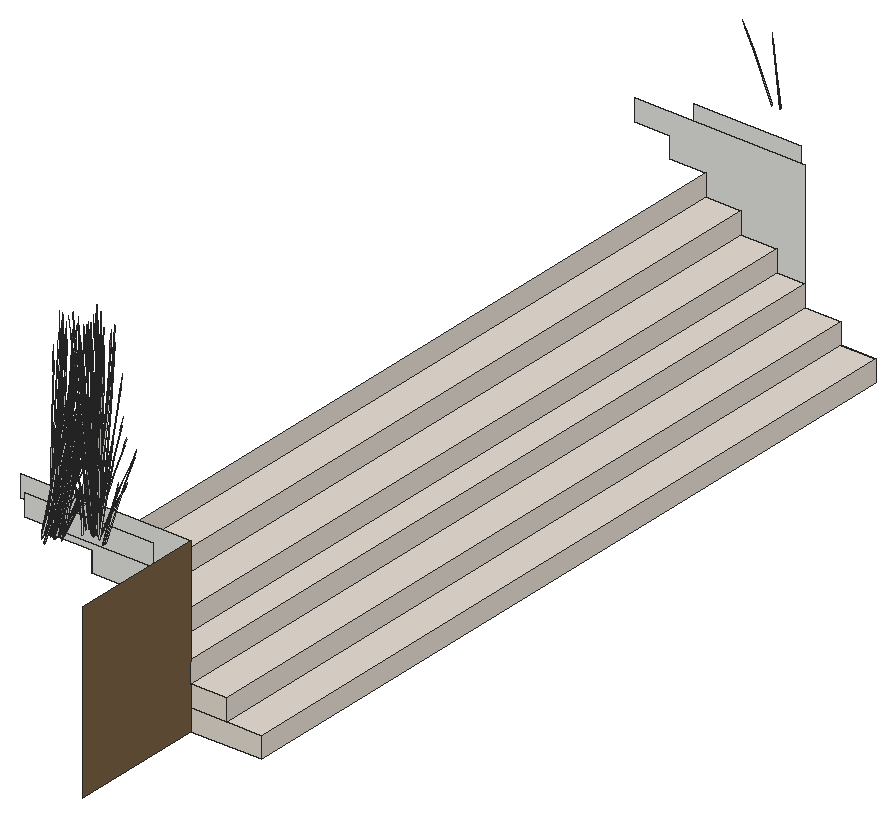
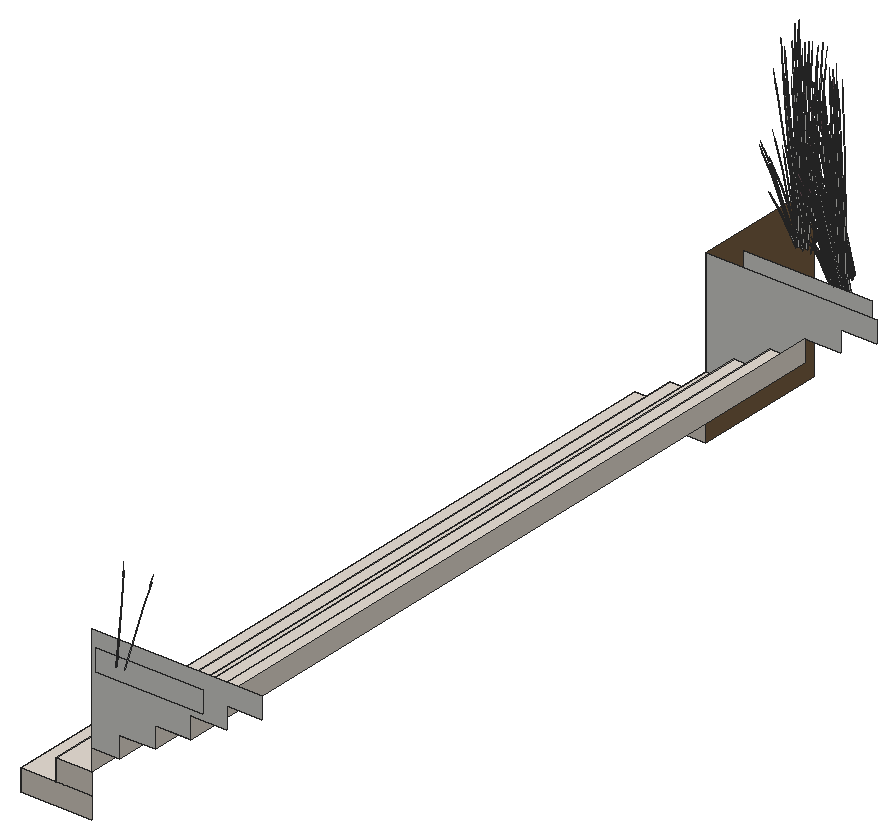
# SketchUp Ruby script. Lengths in inches.
U = 1.inch
M = Sketchup.active_model
def pt(a) = Geom::Point3d.new(a.map { |v| v * U })
def face(e, loops, mat)
  f = e.add_face(loops[0].map { |a| pt(a) })
  loops[1..].each { |l| e.add_face(l.map { |a| pt(a) }).erase! }
  f.material = f.back_material = mat if mat
  f
end
# faces: each face lists its corners as indices into pts; further lists are holes
def faces(e, pts, list, mat = nil) = list.each { |f| face(e, (f[0].is_a?(Array) ? f : [f]).map { |l| l.map { |i| pts[i] } }, mat) }
# xy, xz, yz: faces in a plane at the given z, y or x. An outline is a flat list of corners, or four numbers for a rectangle; further outlines are holes
def ring(l) = l.size == 4 ? [[l[0], l[1]], [l[2], l[1]], [l[2], l[3]], [l[0], l[3]]] : l.each_slice(2).to_a
def flat(e, list, mat, &to3) = list.each { |f| face(e, (f[0].is_a?(Array) ? f : [f]).map { |l| ring(l).map { |u, v| to3.(u, v) } }, mat) }
def xy(e, z, list, mat = nil) = flat(e, list, mat) { |x, y| [x, y, z] }
def xz(e, y, list, mat = nil) = flat(e, list, mat) { |x, z| [x, y, z] }
def yz(e, x, list, mat = nil) = flat(e, list, mat) { |y, z| [x, y, z] }
def lines(e, pts, list) = list.each { |a, b| e.add_line(pt(pts[a]), pt(pts[b])) }
# prism: a flat outline (further loops are holes) pulled along v
def prism(e, loops, v, mat = nil)
  f = face(e, loops, mat); d = Geom::Vector3d.new(v.map { |x| x * U })
  f.pushpull(f.normal.samedirection?(d) ? d.length : -d.length)
end
def box(e, o, s, mat = nil) = prism(e, [[o, [o[0] + s[0], o[1], o[2]], [o[0] + s[0], o[1] + s[1], o[2]], [o[0], o[1] + s[1], o[2]]]], [0, 0, s[2]], mat)
def at(x, y, z, deg = 0) = Geom::Transformation.translation(pt([x, y, z])) * Geom::Transformation.rotation(ORIGIN, Z_AXIS, deg.degrees)
def axes(o, x, y, z) = Geom::Transformation.new([*x, 0, *y, 0, *z, 0, *pt(o).to_a, 1])
def part(name) = M.definitions.add(name)
# library, detail: a bought-in or finely detailed component or shape, given as its bounding box
def library(name, o, s) = part(name).tap { |d| box(d.entities, o, s) }
def detail(e, o, s) = box(e.add_group.entities, o, s)
def put(e, d, t, mat = nil) = e.add_instance(d, t).tap { |i| i.material = mat if mat }
def group(e, t, mat = nil) = e.add_group.tap { |g| g.transformation = t; g.material = mat if mat }.entities
root = M.entities
M.materials.add("LightPink_Translucent").color = [144, 107, 117]
M.materials["LightPink_Translucent"].alpha = 0.75
M.materials.add("Marble_01_1K").color = [230, 221, 211]
M.materials.add("Soil_03_1K").color = [122, 96, 67]
c1 = part("blade")
p = [[2.15,0.21,22],[0,0.17,0],[0.09,0.45,0],[2.18,0.31,22],[2.29,0.31,22],[0.38,0.45,0],
  [2.48,0.24,33],[2.49,0.24,33],[2.48,0.22,33]]
faces(c1.entities,p,[[0,1,2,3],[4,5,2,3],[6,3,4,7],[8,0,3,6]])
c2 = part("seeds")
p = [[0.3,-0.1,1.38],[-0.01,-0.03,1.59],[-0.01,-0.03,0.03],[0.14,-0.07,-0.07],[0.29,-0.03,3],[0.15,0.01,3.11]]
faces(c2.entities,p,[[0,1,2,3],[1,0,4,5]],"LightPink_Translucent")
c3 = part("blade with seeds")
put(c3.entities,c1,at(0,0,0))
put(c3.entities,c2,axes([2.4,0.25,30.99],[1.5799,-0.05474,1.17369],[-0.12525,1.92788,0.29478],[-0.07173,-0.02425,1.56792]))
xy(root,6,[[362,46,372,262]],"Marble_01_1K")
xy(root,12,[[352,46,362,262]],"Marble_01_1K")
xy(root,18,[[344,46,352,262]],"Marble_01_1K")
xy(root,24,[[334,46,344,262]],"Marble_01_1K")
xy(root,30,[[324,46,334,262]],"Marble_01_1K")
xz(root,40,[[310,42,346,48]])
xz(root,46,[[344,18,344,24,334,24,334,30,324,30,324,36,314,36,314,42,304,42,304,48,352,48,352,18]])
xz(root,46,[[352,0,372,6],[352,6,362,12]],"Marble_01_1K")
xz(root,262,[[344,18,352,18,352,48,304,48,304,42,314,42,314,36,324,36,324,30,334,30,334,24,344,24]])
xz(root,262,[[352,0,372,6],[352,6,362,12]],"Marble_01_1K")
xz(root,268,[[316,42,346,48]])
yz(root,324,[[46,30,262,36]],"Marble_01_1K")
yz(root,334,[[46,24,262,30]],"Marble_01_1K")
yz(root,344,[[46,18,262,24]],"Marble_01_1K")
yz(root,352,[[46,12,262,18]],"Marble_01_1K")
yz(root,352,[[8,0,46,48]],"Soil_03_1K")
yz(root,362,[[46,6,262,12]],"Marble_01_1K")
yz(root,372,[[46,0,262,6]],"Marble_01_1K")
put(root,c3,axes([321.74,34.29,43.82],[0.34009,-0.2937,-0.55095],[0.42248,0.26632,-0.1446],[0.13628,-0.07327,1.21613]))
put(root,c3,axes([323.39,30.83,46.18],[-0.22948,0.24822,0.05682],[-0.32679,-0.14452,0.44729],[0.10565,0.07958,0.68204]))
put(root,c3,axes([324.1875,33.59,44.44],[-0.16818,0.19891,1.01491],[-0.14456,-0.26725,0.74569],[0.1389,-0.06697,0.22354]))
put(root,c3,axes([335.68,33.12,50.1875],[0.14586,-0.38834,0.15589],[0.53375,0.1099,0.31002],[-0.0922,0.00189,1.41735]))
put(root,c3,axes([322.85,31.67,46.99],[0.34892,-0.22417,-0.05733],[0.3197,0.24551,-0.25992],[0.02251,0.06957,0.85731]))
put(root,c3,axes([335.56,32.24,49.96],[0.35245,0.2524,0],[-0.35245,0.2524,0],[0,0,1.49564]))
put(root,c3,axes([323.48,30.76,46.18],[-0.5022,0.08967,0.42415],[-0.08716,-0.35177,0.34973],[0.11811,0.10367,0.87768]))
put(root,c3,axes([336.51,32.125,50.1875],[-0.39671,-0.28463,0.15589],[0.39978,-0.27607,0.31002],[-0.04381,0.05813,1.41735]))
put(root,c3,axes([335.78,31.7,49.82],[0.52523,0.06406,-0.55095],[-0.11084,0.39517,-0.1446],[0.15674,0.04788,1.21613]))
put(root,c3,axes([323.95,34.34,46],[0.43951,-0.05584,-0.31292],[0.11606,0.31924,0.40398],[0.12595,-0.08575,0.77298]))
put(root,c3,axes([334.76,33.16,49.94],[-0.50902,-0.17543,0],[0.24498,-0.36452,0],[0,0,1.43768]))
put(root,c3,axes([335.18,32.69,50.18],[-0.49304,-0.31451,-0.2226],[0.41487,-0.35316,0.48713],[-0.13277,0.03679,1.48635]))
put(root,c3,axes([333.89,33.29,50.19],[0.47255,0.19538,0.43871],[-0.28245,0.35034,0],[-0.10763,-0.0445,1.3917]))
put(root,c3,axes([323.26,30.27,44.29],[0.00891,-0.12953,1.26356],[0.4258,-0.14469,-0.27174],[0.13144,0.15503,0.54024]))
put(root,c3,axes([340.42,30.3125,50.29],[0.00891,-0.12953,1.26356],[0.4258,-0.14469,-0.27174],[0.13144,0.15503,0.54024]))
put(root,c3,axes([321.37,34.63,44.36],[-0.05884,-0.44587,-0.25709],[0.6128,-0.02696,-0.44182],[0.10791,-0.05939,1.41118]))
put(root,c3,axes([335.55,31.94,50.4],[0.24498,-0.3521,0.39531],[0.50902,0.16945,-0.19025],[0,0.08116,1.26923]))
put(root,c3,axes([333.95,30.09,50.29],[0.15933,-0.06164,1.26356],[0.39339,0.18587,-0.27174],[-0.11709,0.16083,0.54024]))
put(root,c3,axes([323.59,34.53,46.46],[-0.43951,0.05584,0.31292],[-0.11606,-0.31924,-0.40398],[0.12595,-0.08575,0.77298]))
put(root,c3,axes([322.1,30.72,46.45],[0.49409,-0.18193,-0.10745],[0.24281,0.32289,-0.59638],[0.06519,0.13607,0.90619]))
put(root,c3,axes([335.46,32.14,50.03],[0,0.45191,-0.04981],[-0.63136,0,0],[0,0.0142,1.58489]))
put(root,c3,axes([335.5,31.82,49.95],[0.30332,0.32798,-0.39531],[-0.45944,0.23096,0.19025],[0.09816,0.04058,1.26923]))
put(root,c3,axes([333.61,33.5,50.1],[-0.31568,0.39156,0],[-0.52815,-0.21836,-0.456],[-0.12029,-0.04973,1.44655]))
put(root,c3,axes([321.29,33.64,43.79],[0.47106,0.09668,-0.27372],[-0.11861,0.34048,0.27372],[0.09497,-0.03926,1.22797]))
put(root,c3,axes([336.84,32.14,50.19],[0,-0.39075,0.43871],[0.56491,0,0],[0,0.089,1.3917]))
put(root,c3,axes([335.42,32.43,50.4],[0.54829,-0.02412,0.39531],[0.04958,0.40041,-0.19025],[-0.09816,0.04058,1.26923]))
put(root,c3,axes([339.34,30.84,49.32],[0.08172,-0.02126,1.55816],[0.49154,0.11703,-0.23804],[0.01437,0.1319,0.26541]))
put(root,c3,axes([335.76,32.02,50.3125],[0.47043,-0.11396,0.12794],[0.16474,0.32541,-0.36534],[0,0.07162,1.11991]))
put(root,c3,axes([334.93,32.625,49.95],[-0.54829,0.02412,-0.39531],[-0.04958,-0.40041,0.19025],[-0.09816,0.04058,1.26923]))
put(root,c3,axes([322.53,30.7,46.14],[0.49634,0.09796,-0.45151],[-0.17013,0.33585,-0.34973],[0.04551,0.13522,0.86392]))
put(root,c3,axes([322.81,30.01,45.43],[-0.11542,-0.12546,1.51428],[0.53333,-0.10562,0.12244],[0.12054,0.19696,0.64734]))
put(root,c3,axes([337.51,32.81,50.29],[-0.1216,-0.0961,1.26356],[0.15822,-0.31792,-0.27174],[0.24603,0.04307,0.54024]))
put(root,c3,axes([323.99,34.48,46.18],[0.34663,0.16434,0.05682],[-0.20181,0.23402,0.44729],[0.11113,-0.07566,0.68204]))
put(root,c3,axes([338.21,30.89,50.49],[0.45869,-0.0692,0.0575],[0.10545,0.27878,-0.76259],[-0.02908,0.14112,0.68355]))
put(root,c3,axes([323.89,34.41,46.18],[0.12522,0.35963,0.42415],[-0.49122,0.06241,0.34973],[0.14477,-0.08458,0.87768]))
put(root,c3,axes([325.22,34.84,46.17],[0.07006,-0.05952,1.54581],[-0.08968,-0.3651,-0.24447],[0.1758,-0.06922,0.12397]))
put(root,c3,axes([335.34,33.16,49.95],[0.50902,0.17543,0],[-0.24498,0.36452,0],[0,0,1.54589]))
put(root,c3,axes([335.54,33.55,49.9375],[-0.31175,-0.39292,-0.04544],[0.52815,-0.21836,0.456],[-0.13015,0.03741,1.44584]))
put(root,c3,axes([335.43,32.6,50.3125],[0.37303,0.23477,0.12794],[-0.31115,0.26487,-0.36534],[-0.08661,0.03581,1.11991]))
put(root,c3,axes([322.35,30.64,46.4],[0.24099,0.31773,-0.62776],[-0.49607,0.17707,0.07576],[0.05635,0.15352,0.88802]))
put(root,c3,axes([335.83,33.33,50.19],[0.47255,-0.19538,0.43871],[0.28245,0.35034,0],[-0.10763,0.0445,1.3917]))
put(root,c3,axes([335.16,33.02,50.02],[0.21952,0.44891,-0.05313],[-0.62724,0.1573,0],[0.00767,0.01568,1.52132]))
put(root,c3,axes([335.4,33.5,49.79],[-0.47106,-0.09668,-0.27372],[0.11861,-0.34048,0.27372],[-0.09497,0.03926,1.22797]))
put(root,c3,axes([323.84,35.4,46.45],[-0.25405,-0.35383,-0.10745],[0.45089,-0.17388,-0.59638],[0.19001,-0.04668,0.90619]))
put(root,c3,axes([323.8125,35.09,46.14],[0.13679,-0.35544,-0.45151],[0.46898,0.12183,-0.34973],[0.18882,-0.03259,0.86392]))
put(root,c3,axes([323.07,33.65,44.1],[0.31568,-0.39156,0],[0.52815,0.21836,-0.456],[0.12029,0.04973,1.44655]))
put(root,c3,axes([332,32.8125,50.29],[0.17547,0.03208,1.26356],[0.1131,0.32764,-0.27174],[-0.23835,0.06133,0.54024]))
put(root,c3,axes([338.1,31.1875,50.29],[0.15933,-0.06164,1.26356],[0.39339,0.18587,-0.27174],[-0.11709,0.16083,0.54024]))
put(root,c3,axes([321.99,31.44,46.17],[0.064,0.06292,1.54581],[0.51651,0.02472,-0.24447],[0.05194,0.13877,0.12397]))
put(root,c3,axes([337.22,32.2,50.1],[0.63136,0,0],[0,0.43672,-0.456],[0,0.09947,1.44655]))
put(root,c3,axes([336.97,32.43,49.94],[-0.63105,-0.00312,-0.04397],[0,-0.43672,0.44129],[-0.01983,0.09942,1.3992]))
put(root,c3,axes([335.6,32.05,50.36],[0.56863,0.18645,-0.25709],[-0.2738,0.39352,-0.44182],[0.01787,0.09662,1.41118]))
put(root,c3,axes([324.32,35.19,43.75],[-0.3252,0.04689,1.25103],[-0.05176,-0.37326,0.07161],[0.22777,-0.0565,0.71188]))
put(root,c3,axes([324.91,34.86,44],[-0.31304,-0.24986,-0.05733],[0.34284,-0.22894,-0.25992],[0.09714,-0.01612,0.85731]))
put(root,c3,axes([336.84,32.49,49.79],[-0.35245,0.2438,-0.27372],[-0.35245,-0.2438,0.27372],[0,0.07853,1.22797]))
put(root,c3,axes([335.32,32.52,50.36],[0.05884,0.44587,-0.25709],[-0.6128,0.02696,-0.44182],[-0.10791,0.05939,1.41118]))
put(root,c3,axes([335.54,32.34,49.95],[-0.24498,0.3521,-0.39531],[-0.50902,-0.16945,0.19025],[0,0.08116,1.26923]))
put(root,c3,axes([322.8,33.85,44.19],[-0.47255,-0.19538,0.43871],[0.28245,-0.35034,0],[0.10763,0.0445,1.3917]))
put(root,c3,axes([323.72,35.22,46.4],[0.44368,-0.17257,-0.62776],[0.24726,0.35524,0.07576],[0.21437,-0.04035,0.88802]))
put(root,c3,axes([321.74,34.61,44.09],[-0.41865,0.35461,0.40429],[-0.49737,-0.31303,0.15865],[0.10093,-0.03539,1.40366]))
put(root,c3,axes([323.66,35.29,46.46],[-0.41962,-0.10901,0.31292],[0.12239,-0.31802,-0.40398],[0.16894,-0.02916,0.77298]))
put(root,c3,axes([334.95,32.86,49.82],[-0.34009,0.2937,-0.55095],[-0.42248,-0.26632,-0.1446],[-0.13628,0.07327,1.21613]))
put(root,c3,axes([320.79,34.34,43.41],[-0.49699,0.15644,1.13921],[-0.15819,-0.44887,0.44265],[0.30518,0.00747,1.29573]))
put(root,c3,axes([322.125,34.46,44.3125],[0.09741,-0.34873,0.12794],[0.4759,0.06053,-0.36534],[0.08661,0.03581,1.11991]))
put(root,c3,axes([335.55,33.35,50.06],[0.63212,0.12701,0.27176],[-0.15814,0.45398,-0.32244],[-0.10462,0.05682,1.45692]))
put(root,c3,axes([335.51,33.66,49.78],[-0.47255,0.19538,-0.43871],[-0.28245,-0.35034,0],[-0.10763,0.0445,1.3917]))
put(root,c3,axes([337.08,32.5,49.78],[0,0.39075,-0.43871],[-0.56491,0,0],[0,0.089,1.3917]))
put(root,c3,axes([324.67,34.95,43.32],[-0.02639,-0.05932,1.55816],[0.18302,-0.34702,-0.23804],[0.18462,-0.00499,0.26541]))
put(root,c3,axes([321.92,34.55,44.4],[-0.30332,-0.32798,0.39531],[0.45944,-0.23096,-0.19025],[0.09816,0.04058,1.26923]))
put(root,c3,axes([322.08,34.57,44.36],[0.50979,-0.25942,-0.25709],[0.339,0.36656,-0.44182],[0.12578,0.03723,1.41118]))
put(root,c3,axes([324.1,35.25,46],[0.41962,0.10901,-0.31292],[-0.12239,0.31802,0.40398],[0.16894,-0.02916,0.77298]))
put(root,c3,axes([323.36,33.88,43.78],[0.47255,0.19538,-0.43871],[-0.28245,0.35034,0],[0.10763,0.0445,1.3917]))
put(root,c3,axes([322.46,35,43.95],[0.56491,0,0],[0,0.40454,0],[0,0,1.5764]))
put(root,c3,axes([335.9375,33.6,50.1],[0.31568,0.39156,0],[-0.52815,0.21836,-0.456],[-0.12029,0.04973,1.44655]))
put(root,c3,axes([336.44,33.73,49.32],[0.03679,-0.05641,1.55816],[0.46313,-0.16615,-0.23804],[0.14041,0.08599,0.26541]))
put(root,c3,axes([335.83,32.45,49.85],[0.18514,0.35777,-0.61156],[-0.53331,0.12885,-0.16051],[0.02046,0.12115,1.3499]))
put(root,c3,axes([332.1875,33.68,49.32],[0.06773,0.03904,1.55816],[0.11484,0.36171,-0.23804],[-0.15011,0.07713,0.26541]))
put(root,c3,axes([322.96,34.86,45.43],[-0.20943,0.00885,1.51428],[0.13893,-0.38357,0.12244],[0.29846,0.02372,0.64734]))
put(root,c3,axes([323.23,34.03,43.79],[0.11861,0.34048,-0.27372],[-0.47106,0.09668,0.27372],[0.09497,0.03926,1.22797]))
put(root,c3,axes([324.04,35.39,46.18],[0.18545,0.26643,0.05682],[-0.33817,0.13041,0.44729],[0.14907,-0.02573,0.68204]))
put(root,c3,axes([322.28,34.79,44.1],[-0.63817,-0.08233,0.43472],[0.12987,-0.46497,0.17059],[0.09326,0.0449,1.50931]))
put(root,c3,axes([324,35.29,46.18],[-0.14265,0.35629,0.42415],[-0.46898,-0.12183,0.34973],[0.18443,-0.02141,0.87768]))
put(root,c3,axes([336.41,33.82,50.36],[-0.32378,-0.01225,0.92831],[0.21383,-0.26028,0.51254],[0.12791,0.09247,0.72818]))
put(root,c3,axes([322.39,35.89,43.93],[0.53009,-0.13258,-0.16963],[0.18627,0.38191,0.00007],[0.05851,-0.01465,1.53656]))
put(root,c3,axes([322.45,35.17,43.96],[0.35245,0.2524,0],[-0.35245,0.2524,0],[0,0,1.49564]))
put(root,c3,axes([322.67,34.63,43.82],[0.52523,0.06406,-0.55095],[-0.11084,0.39517,-0.1446],[0.15674,0.04788,1.21613]))
put(root,c3,axes([324.99,35.32,44.44],[-0.31197,0.06451,1.01491],[0.14684,-0.26661,0.74569],[0.1655,0.01824,0.22354]))
put(root,c3,axes([335.35,33.19,50.29],[0.00891,-0.12953,1.26356],[0.4258,-0.14469,-0.27174],[0.13144,0.15503,0.54024]))
put(root,c3,axes([322.45,34.875,44.4],[0.24498,-0.3521,0.39531],[0.50902,0.16945,-0.19025],[0,0.08116,1.26923]))
put(root,c3,axes([324.85,36.45,46.16],[-0.04566,-0.03421,1.56736],[0.09987,-0.36669,-0.1481],[0.17984,-0.02343,0.27737]))
put(root,c3,axes([322.4,34.75,43.95],[0.30332,0.32798,-0.39531],[-0.45944,0.23096,0.19025],[0.09816,0.04058,1.26923]))
put(root,c3,axes([324.45,36.14,45.47],[-0.09664,-0.32847,-0.03085],[0.45676,-0.07551,-0.13989],[0.09538,0.02082,0.4614]))
put(root,c3,axes([323.27,36.13,46.45],[0.02704,-0.39739,-0.10745],[0.51189,0.01086,-0.59638],[0.19715,0.0276,0.90619]))
put(root,c3,axes([334.28,33.72,49.32],[0.08172,-0.02126,1.55816],[0.49154,0.11703,-0.23804],[0.01437,0.1319,0.26541]))
put(root,c3,axes([323.73,35.07,44.19],[0,-0.39075,0.43871],[0.56491,0,0],[0,0.089,1.3917]))
put(root,c3,axes([322.66,34.95,44.3125],[0.47043,-0.11396,0.12794],[0.16474,0.32541,-0.36534],[0,0.07162,1.11991]))
put(root,c3,axes([323.1875,35.98,46.46],[-0.28729,-0.24465,0.31292],[0.32804,-0.23159,-0.40398],[0.16667,0.03524,0.77298]))
put(root,c3,axes([333.15,33.77,50.49],[0.45869,-0.0692,0.0575],[0.10545,0.27878,-0.76259],[-0.02908,0.14112,0.68355]))
put(root,c3,axes([324.41,35.75,44.29],[-0.1216,-0.0961,1.26356],[0.15822,-0.31792,-0.27174],[0.24603,0.04307,0.54024]))
put(root,c3,axes([322.23,36.1,43.95],[0.50902,0.17543,0],[-0.24498,0.36452,0],[0,0,1.54589]))
put(root,c3,axes([323.71,35.89,46.17],[0.10831,-0.00661,1.54581],[0.29709,-0.30358,-0.24447],[0.19266,0.04007,0.12397]))
put(root,c3,axes([323.29,35.94,46.4],[0.50473,0.00941,-0.62776],[-0.0339,0.39618,0.07576],[0.21383,0.04181,0.88802]))
put(root,c3,axes([333.04,34.06,50.29],[0.15933,-0.06164,1.26356],[0.39339,0.18587,-0.27174],[-0.11709,0.16083,0.54024]))
put(root,c3,axes([324.12,35.14,44.1],[0.63136,0,0],[0,0.43672,-0.456],[0,0.09947,1.44655]))
put(root,c3,axes([322.5,34.98,44.36],[0.56863,0.18645,-0.25709],[-0.2738,0.39352,-0.44182],[0.01787,0.09662,1.41118]))
put(root,c3,axes([323.59,36.1,46],[0.28729,0.24465,-0.31292],[-0.32804,0.23159,0.40398],[0.16667,0.03524,0.77298]))
put(root,c3,axes([323.73,35.42,43.79],[-0.35245,0.2438,-0.27372],[-0.35245,-0.2438,0.27372],[0,0.07853,1.22797]))
put(root,c3,axes([323.45,36.2,46.18],[-0.02542,0.29714,0.05682],[-0.38391,-0.00815,0.44729],[0.14706,0.03109,0.68204]))
put(root,c3,axes([323.48,36.1,46.18],[-0.3723,0.25748,0.42415],[-0.32109,-0.27343,0.34973],[0.17467,0.04749,0.87768]))
put(root,c3,axes([322.3,36.4,46.46],[-0.07798,-0.31474,0.31292],[0.44579,-0.08311,-0.40398],[0.11974,0.09019,0.77298]))
put(root,c3,axes([323.97,35.43,43.78],[0,0.39075,-0.43871],[-0.56491,0,0],[0,0.089,1.3917]))
put(root,c3,axes([322.5625,35.48,45.43],[-0.18755,-0.06732,1.51428],[0.38813,-0.28243,0.12244],[0.24191,0.12741,0.64734]))
put(root,c3,axes([322.6,34.59,45.95],[-0.4363,-0.20303,1.22187],[0.46069,-0.31611,0.5272],[0.14077,0.1905,1.18105]))
put(root,c3,axes([323.26,36.24,44.44],[-0.28429,-0.11236,1.01491],[0.36709,-0.11416,0.74569],[0.09901,0.0967,0.22354]))
put(root,c3,axes([322.26,36.5625,46.45],[0.30087,-0.33447,-0.10745],[0.43572,0.19269,-0.59638],[0.15146,0.0945,0.90619]))
put(root,c3,axes([321.86,36.84,46.16],[0.00149,-0.04731,1.56736],[0.4327,-0.20872,-0.1481],[0.1503,0.0745,0.27737]))
put(root,c3,axes([323.34,36.66,43.32],[0.03679,-0.05641,1.55816],[0.46313,-0.16615,-0.23804],[0.14041,0.08599,0.26541]))
put(root,c3,axes([322.73,35.38,43.85],[0.18514,0.35777,-0.61156],[-0.53331,0.12885,-0.16051],[0.02046,0.12115,1.3499]))
put(root,c3,axes([322.61,36.4,46.14],[0.49824,-0.09289,-0.45151],[0.08716,0.35177,-0.34973],[0.13382,0.10081,0.86392]))
put(root,c3,axes([323.3,36.75,44.36],[-0.32378,-0.01225,0.92831],[0.21383,-0.26028,0.51254],[0.12791,0.09247,0.72818]))
put(root,c3,axes([322.37,36.6875,46.18],[-0.22948,0.24822,0.05682],[-0.32679,-0.14452,0.44729],[0.10565,0.07958,0.68204]))
put(root,c3,axes([321.83,37.52,46.99],[0.34892,-0.22417,-0.05733],[0.3197,0.24551,-0.25992],[0.02251,0.06957,0.85731]))
put(root,c3,axes([322.47,36.62,46.18],[-0.5022,0.08967,0.42415],[-0.08716,-0.35177,0.34973],[0.11811,0.10367,0.87768]))
put(root,c3,axes([322.25,36.125,44.29],[0.00891,-0.12953,1.26356],[0.4258,-0.14469,-0.27174],[0.13144,0.15503,0.54024]))
put(root,c3,axes([321.08,36.58,46.45],[0.49409,-0.18193,-0.10745],[0.24281,0.32289,-0.59638],[0.06519,0.13607,0.90619]))
put(root,c3,axes([321.51,36.5625,46.14],[0.49634,0.09796,-0.45151],[-0.17013,0.33585,-0.34973],[0.04551,0.13522,0.86392]))
put(root,c3,axes([321.79,35.87,45.43],[-0.11542,-0.12546,1.51428],[0.53333,-0.10562,0.12244],[0.12054,0.19696,0.64734]))
put(root,c3,axes([334.77,274.96,50.29],[-0.14352,0.07909,1.26356],[-0.42983,-0.13843,-0.27174],[0.07968,-0.17216,0.54024]))
put(root,c3,axes([332.55,274.81,50.29],[-0.03058,0.12783,1.26356],[-0.44698,0.10701,-0.27174],[-0.10448,-0.16522,0.54024]))
